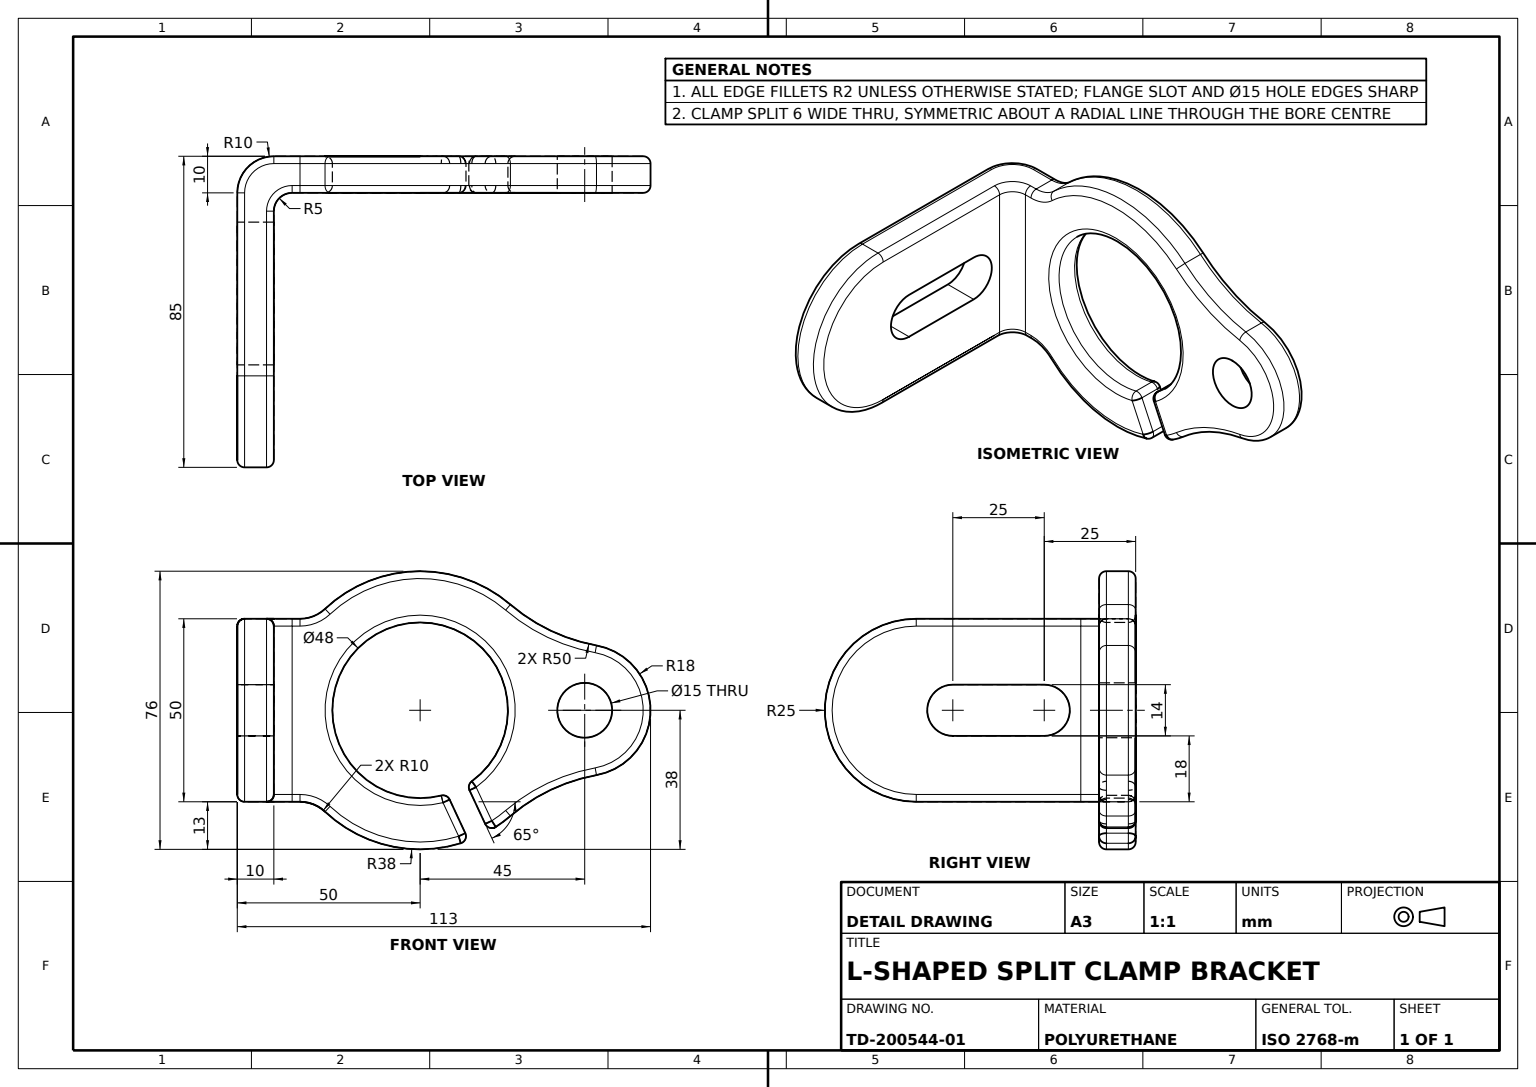
solid
v1 (-28.889805,-74.685606,8)
v2 (-28.889805,-74.685606,2)
e1 v1 v2 LINE
v3 (-38,-50,8)
e2 v1 v3 CIRCLE(AX(P(0,-50,8),D(0,0,-1),D(1,0,0)),38)
v4 (-38,-50,2)
e3 v3 v4 LINE
e4 v4 v2 CIRCLE(AX(P(0,-50,2),D(0,0,1),D(1,0,0)),38)
face CYL(AX(P(0,-50,10),D(0,0,-1),D(-1,0,0)),38) [-e1 e2 e3 e4]
v5 (-23,-10,-50)
v6 (-25,-8,-50)
e5 v5 v6 CIRCLE(AX(P(-23,-8,-50),D(0,0,-1),D(-1,0,0)),2)
v7 (25,-8,-50)
e6 v7 v6 CIRCLE(AX(P(0,-8,-50),D(0,1,0),D(1,0,0)),25)
v8 (23,-10,-50)
e7 v8 v7 CIRCLE(AX(P(23,-8,-50),D(0,0,1),D(1,0,0)),2)
e8 v5 v8 CIRCLE(AX(P(0,-10,-50),D(0,-1,0),D(1,0,0)),23)
face TORUS(AX(P(0,-8,-50),D(0,-1,0),D(1,0,0)),23,2) [e5 -e6 -e7 -e8]
v9 (26,-50,10)
v10 (24,-50,8)
e9 v9 v10 CIRCLE(AX(P(26,-50,8),D(0,-1,0),D(0,0,-1)),2)
v11 (-26,-50,10)
e10 v11 v9 CIRCLE(AX(P(0,-50,10),D(0,0,-1),D(1,0,0)),26)
v12 (-24,-50,8)
e11 v11 v12 CIRCLE(AX(P(-26,-50,8),D(0,1,0),D(-1,0,0)),2)
e12 v10 v12 CIRCLE(AX(P(0,-50,8),D(0,0,1),D(1,0,0)),24)
face TORUS(AX(P(0,-50,8),D(0,0,1),D(1,0,0)),26,2) [-e9 -e10 e11 -e12]
v13 (23.295936,-55.77056,2)
v14 (23.237264,-56.25144,2)
e13 v13 v14 CIRCLE(AX(P(25.237264,-56.25144,2),D(0,0,1),D(-1,0,0)),2)
v15 (23.237264,-56.25144,8)
e14 v15 v14 LINE
v16 (23.295936,-55.77056,8)
e15 v16 v15 CIRCLE(AX(P(25.237264,-56.25144,8),D(0,0,1),D(1,0,0)),2)
e16 v13 v16 LINE
face CYL(AX(P(25.237264,-56.25144,10),D(0,0,-1),D(-1,0,0)),2) [e13 -e14 -e15 -e16]
v17 (-25,-2,-50)
v18 (25,-2,-50)
e17 v17 v18 CIRCLE(AX(P(0,-2,-50),D(0,-1,0),D(1,0,0)),25)
v19 (-23,0,-50)
e18 v19 v17 CIRCLE(AX(P(-23,-2,-50),D(0,0,1),D(1,0,0)),2)
v20 (23,0,-50)
e19 v20 v19 CIRCLE(AX(P(0,0,-50),D(0,1,0),D(1,0,0)),23)
e20 v20 v18 CIRCLE(AX(P(23,-2,-50),D(0,0,-1),D(-1,0,0)),2)
face TORUS(AX(P(0,-2,-50),D(0,-1,0),D(1,0,0)),23,2) [-e17 -e18 -e19 e20]
v21 (-7.5,-95,0)
v22 (7.5,-95,0)
e21 v21 v22 CIRCLE(AX(P(0,-95,0),D(0,0,1),D(1,0,0)),7.5)
v23 (-7.5,-95,10)
e22 v23 v21 LINE
v24 (7.5,-95,10)
e23 v23 v24 CIRCLE(AX(P(0,-95,10),D(0,0,1),D(1,0,0)),7.5)
e24 v24 v22 LINE
face CYL(AX(P(0,-95,10),D(0,0,-1),D(-1,0,0)),7.5) rev [-e21 -e22 e23 e24]
v25 (17.70954,-98.220588,8)
v26 (15.741813,-97.862745,10)
e25 v25 v26 CIRCLE(AX(P(15.741813,-97.862745,8),D(-0.178921569,-0.98386334,0),D(0.98386334,-0.178921569,0)),2)
v27 (-15.741813,-97.862745,10)
e26 v27 v26 CIRCLE(AX(P(0,-95,10),D(0,0,1),D(1,0,0)),16)
v28 (-17.70954,-98.220588,8)
e27 v28 v27 CIRCLE(AX(P(-15.741813,-97.862745,8),D(-0.178921569,0.98386334,0),D(-0.98386334,-0.178921569,0)),2)
e28 v25 v28 CIRCLE(AX(P(0,-95,8),D(0,0,-1),D(1,0,0)),18)
face TORUS(AX(P(0,-95,8),D(0,0,1),D(1,0,0)),16,2) [e25 -e26 -e27 -e28]
v29 (23,-10,10)
v30 (-23,-10,10)
e29 v29 v30 LINE
v31 (23,0,0)
e30 v29 v31 CIRCLE(AX(P(23,-10,0),D(-1,0,0),D(0,-1,0)),10)
v32 (-23,0,0)
e31 v32 v31 LINE
e32 v32 v30 CIRCLE(AX(P(-23,-10,0),D(1,0,0),D(0,1,0)),10)
face CYL(AX(P(-66.902707,-10,0),D(1,0,0),D(0,1,0)),10) [-e29 e30 -e31 e32]
v33 (28.889805,-74.685606,2)
v34 (27.369289,-73.386364,0)
e33 v33 v34 CIRCLE(AX(P(27.369289,-73.386364,2),D(0.649621212,0.760258036,0),D(-0.760258036,0.649621212,0)),2)
v35 (17.70954,-98.220588,2)
e34 v35 v33 CIRCLE(AX(P(66.902707,-107.166667,2),D(0,0,-1),D(1,0,0)),50)
v36 (15.741813,-97.862745,0)
e35 v35 v36 CIRCLE(AX(P(15.741813,-97.862745,2),D(0.178921569,0.98386334,0),D(-0.98386334,0.178921569,0)),2)
e36 v34 v36 CIRCLE(AX(P(66.902707,-107.166667,0),D(0,0,1),D(1,0,0)),52)
face TORUS(AX(P(66.902707,-107.166667,2),D(0,0,1),D(1,0,0)),52,2) [-e33 -e34 e35 -e36]
v37 (19.394844,-64.136478,8)
v38 (19.394844,-64.136478,2)
e37 v37 v38 LINE
v39 (21.856318,-63.501902,8)
e38 v39 v37 CIRCLE(AX(P(21.011081,-65.314518,8),D(0,0,1),D(1,0,0)),2)
v40 (21.856318,-63.501902,2)
e39 v40 v39 LINE
v41 (21.011081,-63.314518,2)
e40 v40 v41 CIRCLE(AX(P(21.011081,-65.314518,2),D(0,0,1),D(-1,0,0)),2)
e41 v41 v38 CIRCLE(AX(P(21.011081,-65.314518,2),D(0,0,1),D(-1,0,0)),2)
face CYL(AX(P(21.011081,-65.314518,10),D(0,0,-1),D(-1,0,0)),2) [-e37 -e38 -e39 e40 e41]
v42 (-25,-10,8)
e42 v30 v42 CIRCLE(AX(P(-23,-10,8),D(0,-1,0),D(0,0,-1)),2)
v43 (-25,-17.151865,8)
e43 v43 v42 LINE
v44 (-23,-17.151865,10)
e44 v43 v44 CIRCLE(AX(P(-23,-17.151865,8),D(0,1,0),D(0,0,1)),2)
e45 v30 v44 LINE
face CYL(AX(P(-23,-107.166667,8),D(0,1,0),D(-1,0,0)),2) [e42 -e43 e44 -e45]
v45 (-17.70954,-98.220588,2)
e46 v45 v35 CIRCLE(AX(P(0,-95,2),D(0,0,1),D(1,0,0)),18)
v46 (-15.741813,-97.862745,0)
e47 v45 v46 CIRCLE(AX(P(-15.741813,-97.862745,2),D(0.178921569,-0.98386334,0),D(0.98386334,0.178921569,0)),2)
e48 v36 v46 CIRCLE(AX(P(0,-95,0),D(0,0,-1),D(1,0,0)),16)
face TORUS(AX(P(0,-95,2),D(0,0,1),D(1,0,0)),16,2) [-e46 e47 -e48 -e35]
v47 (31.87542,-70.687136,2)
v48 (30.197766,-69.598339,0)
e49 v47 v48 CIRCLE(AX(P(30.197766,-69.598339,2),D(0.544398315,0.838826844,0),D(-0.838826844,0.544398315,0)),2)
v49 (31.043003,-67.785724,2)
e50 v48 v49 CIRCLE(AX(P(30.197766,-69.598339,2),D(0.906307787,-0.422618262,0),D(0.422618262,0.906307787,0)),2)
e51 v47 v49 CIRCLE(AX(P(30.197766,-69.598339,2),D(0,0,1),D(-1,0,0)),2)
face SPHERE(AX(P(30.197766,-69.598339,2),D(0,1,0),D(-1,0,0)),2) [e49 e50 -e51]
v50 (-25,-2,0)
e52 v50 v17 LINE
e53 v32 v50 CIRCLE(AX(P(-23,-2,0),D(0,0,1),D(1,0,0)),2)
e54 v19 v32 LINE
face CYL(AX(P(-23,-2,10),D(0,0,-1),D(-1,0,0)),2) [-e52 -e53 -e54 e18]
e55 v33 v47 CIRCLE(AX(P(0,-50,2),D(0,0,1),D(1,0,0)),38)
e56 v48 v34 CIRCLE(AX(P(0,-50,0),D(0,0,-1),D(1,0,0)),36)
face TORUS(AX(P(0,-50,2),D(0,0,1),D(1,0,0)),36,2) [-e55 e33 -e56 -e49]
v51 (7,-10,-40)
v52 (7,0,-40)
e57 v51 v52 LINE
v53 (-7,0,-40)
e58 v52 v53 CIRCLE(AX(P(0,0,-40),D(0,1,0),D(-1,0,0)),7)
v54 (-7,-10,-40)
e59 v54 v53 LINE
e60 v51 v54 CIRCLE(AX(P(0,-10,-40),D(0,1,0),D(-1,0,0)),7)
face CYL(AX(P(0,-10,-40),D(0,1,0),D(-1,0,0)),7) rev [e57 e58 -e59 -e60]
v55 (-24,-50,2)
e61 v38 v55 CIRCLE(AX(P(0,-50,2),D(0,0,-1),D(1,0,0)),24)
e62 v12 v55 LINE
e63 v12 v37 CIRCLE(AX(P(0,-50,8),D(0,0,1),D(1,0,0)),24)
face CYL(AX(P(0,-50,10),D(0,0,-1),D(-1,0,0)),24) rev [e61 -e62 e63 e37]
v56 (7,-10,-15)
e64 v56 v51 LINE
v57 (7,0,-15)
e65 v56 v57 LINE
e66 v57 v52 LINE
face PLANE(AX(P(7,-10,-40),D(1,0,0),D(0,0,-1))) rev [-e64 e65 e66 -e57]
v58 (25.237264,-56.25144,10)
v59 (24.392028,-58.064055,8)
e67 v58 v59 CIRCLE(AX(P(25.237264,-56.25144,8),D(0.906307787,-0.422618262,0),D(-0.422618262,-0.906307787,0)),2)
e68 v16 v58 CIRCLE(AX(P(25.237264,-56.25144,8),D(0.240439997,0.970664004,0),D(0.970664004,-0.240439997,0)),2)
e69 v15 v59 CIRCLE(AX(P(25.237264,-56.25144,8),D(0,0,1),D(1,0,0)),2)
face SPHERE(AX(P(25.237264,-56.25144,8),D(1,0,0),D(0,-1,0)),2) [-e67 -e68 e15 e69]
v60 (23,-10,-5)
e70 v8 v60 LINE
v61 (25,-8,-5)
e71 v61 v7 LINE
e72 v60 v61 CIRCLE(AX(P(23,-8,-5),D(0,0,1),D(1,0,0)),2)
face CYL(AX(P(23,-8,10),D(0,0,1),D(1,0,0)),2) [-e70 e7 -e71 -e72]
v62 (25,-17.151865,8)
v63 (27.708333,-23.995226,8)
e73 v62 v63 CIRCLE(AX(P(35,-17.151865,8),D(0,0,1),D(1,0,0)),10)
v64 (23,-17.151865,10)
e74 v64 v62 CIRCLE(AX(P(23,-17.151865,8),D(0,1,0),D(0,0,1)),2)
v65 (26.25,-25.363898,10)
e75 v65 v64 CIRCLE(AX(P(35,-17.151865,10),D(0,0,-1),D(1,0,0)),12)
e76 v65 v63 CIRCLE(AX(P(26.25,-25.363898,8),D(-0.684336154,0.729166667,0),D(-0.729166667,-0.684336154,0)),2)
face TORUS(AX(P(35,-17.151865,8),D(0,0,1),D(1,0,0)),12,2) [-e73 -e74 -e75 e76]
e77 v28 v45 LINE
e78 v25 v35 LINE
face CYL(AX(P(0,-95,10),D(0,0,-1),D(-1,0,0)),18) [e28 e77 e46 -e78]
v66 (-7,-10,-15)
e79 v54 v66 LINE
e80 v66 v56 CIRCLE(AX(P(0,-10,-15),D(0,1,0),D(-1,0,0)),7)
v67 (-23,-10,-5)
e81 v67 v5 LINE
e82 v60 v67 LINE
face PLANE(AX(P(0,-10,-50),D(0,-1,0),D(1,0,0))) [e79 e80 e64 e60] [e81 e8 e70 e82]
e83 v42 v50 CIRCLE(AX(P(-25,-10,0),D(-1,0,0),D(0,1,0)),8)
e84 v6 v17 LINE
v68 (-25,-8,-5)
e85 v6 v68 LINE
v69 (-25,-15,2)
e86 v68 v69 CIRCLE(AX(P(-25,-15,-5),D(1,0,0),D(0,1,0)),7)
v70 (-25,-17.151865,2)
e87 v69 v70 LINE
e88 v43 v70 LINE
face PLANE(AX(P(-25,0,10),D(1,0,0),D(0,1,0))) rev [e43 e83 e52 -e84 e85 e86 e87 -e88]
v71 (24,-50,2)
e89 v71 v13 CIRCLE(AX(P(0,-50,2),D(0,0,-1),D(1,0,0)),24)
e90 v16 v10 CIRCLE(AX(P(0,-50,8),D(0,0,1),D(1,0,0)),24)
e91 v10 v71 LINE
face CYL(AX(P(0,-50,10),D(0,0,-1),D(-1,0,0)),24) rev [e89 e16 e90 e91]
v72 (25,-2,0)
e92 v18 v72 LINE
v73 (25,-10,8)
e93 v72 v73 CIRCLE(AX(P(25,-10,0),D(1,0,0),D(0,-1,0)),8)
e94 v73 v62 LINE
v74 (25,-17.151865,2)
e95 v62 v74 LINE
v75 (25,-15,2)
e96 v74 v75 LINE
e97 v75 v61 CIRCLE(AX(P(25,-15,-5),D(-1,0,0),D(0,-1,0)),7)
e98 v7 v18 LINE
face PLANE(AX(P(25,0,10),D(-1,0,0),D(0,-1,0))) rev [e92 e93 e94 e95 e96 e97 e71 e98]
e99 v9 v58 CIRCLE(AX(P(0,-50,10),D(0,0,-1),D(1,0,0)),26)
face TORUS(AX(P(0,-50,8),D(0,0,1),D(1,0,0)),26,2) [e68 -e99 e9 -e90]
v76 (31.043003,-67.785724,8)
e100 v39 v76 LINE
e101 v76 v49 LINE
e102 v49 v40 LINE
face PLANE(AX(P(35.208422,-69.728091,10),D(-0.422618262,-0.906307787,0),D(0.906307787,-0.422618262,0))) rev [e39 e100 e101 e102]
e103 v29 v73 CIRCLE(AX(P(23,-10,8),D(0,1,0),D(0,0,1)),2)
e104 v64 v29 LINE
face CYL(AX(P(23,-107.166667,8),D(0,-1,0),D(1,0,0)),2) [e74 -e94 -e103 -e104]
v77 (-27.369289,-73.386364,10)
e105 v1 v77 CIRCLE(AX(P(-27.369289,-73.386364,8),D(-0.649621212,0.760258036,0),D(-0.760258036,-0.649621212,0)),2)
e106 v28 v1 CIRCLE(AX(P(-66.902707,-107.166667,8),D(0,0,1),D(1,0,0)),50)
e107 v77 v27 CIRCLE(AX(P(-66.902707,-107.166667,10),D(0,0,-1),D(1,0,0)),52)
face TORUS(AX(P(-66.902707,-107.166667,8),D(0,0,1),D(1,0,0)),52,2) [-e105 -e106 e27 -e107]
e108 v55 v71 CIRCLE(AX(P(0,-50,2),D(0,0,-1),D(1,0,0)),24)
v78 (-26,-50,0)
e109 v55 v78 CIRCLE(AX(P(-26,-50,2),D(0,1,0),D(-1,0,0)),2)
v79 (26,-50,0)
e110 v79 v78 CIRCLE(AX(P(0,-50,0),D(0,0,1),D(1,0,0)),26)
e111 v71 v79 CIRCLE(AX(P(26,-50,2),D(0,-1,0),D(0,0,-1)),2)
face TORUS(AX(P(0,-50,2),D(0,0,1),D(1,0,0)),26,2) [-e108 e109 -e110 -e111]
e112 v24 v23 CIRCLE(AX(P(0,-95,10),D(0,0,1),D(1,0,0)),7.5)
v80 (-26.25,-25.363898,10)
e113 v44 v80 CIRCLE(AX(P(-35,-17.151865,10),D(0,0,-1),D(1,0,0)),12)
e114 v80 v77 CIRCLE(AX(P(0,-50,10),D(0,0,1),D(1,0,0)),36)
v81 (27.369289,-73.386364,10)
e115 v26 v81 CIRCLE(AX(P(66.902707,-107.166667,10),D(0,0,-1),D(1,0,0)),52)
v82 (30.197766,-69.598339,10)
e116 v81 v82 CIRCLE(AX(P(0,-50,10),D(0,0,1),D(1,0,0)),36)
v83 (21.011081,-65.314518,10)
e117 v82 v83 LINE
e118 v83 v11 CIRCLE(AX(P(0,-50,10),D(0,0,-1),D(1,0,0)),26)
v84 (34.423949,-60.535261,10)
e119 v58 v84 LINE
v85 (36,-50,10)
e120 v84 v85 CIRCLE(AX(P(0,-50,10),D(0,0,1),D(1,0,0)),36)
e121 v85 v65 CIRCLE(AX(P(0,-50,10),D(0,0,1),D(1,0,0)),36)
face PLANE(AX(P(-66.902707,-107.166667,10),D(0,0,1),D(1,0,0))) [-e23 -e112] [e45 e113 e114 e107 e26 e115 e116 e117 e118 e10 e99 e119 e120 e121 e75 e104 e29]
v86 (31.87542,-70.687136,8)
e122 v86 v76 CIRCLE(AX(P(30.197766,-69.598339,8),D(0,0,1),D(1,0,0)),2)
e123 v76 v82 CIRCLE(AX(P(30.197766,-69.598339,8),D(0.906307787,-0.422618262,0),D(0.422618262,0.906307787,0)),2)
e124 v86 v82 CIRCLE(AX(P(30.197766,-69.598339,8),D(-0.544398315,-0.838826844,0),D(-0.838826844,0.544398315,0)),2)
face SPHERE(AX(P(30.197766,-69.598339,8),D(1,0,0),D(0,-1,0)),2) [e122 e123 -e124]
e125 v47 v86 LINE
face CYL(AX(P(30.197766,-69.598339,10),D(0,0,-1),D(-1,0,0)),2) [-e101 -e122 -e125 e51]
v87 (24.392028,-58.064055,2)
v88 (33.578712,-62.347877,2)
e126 v87 v88 LINE
v89 (33.578712,-62.347877,8)
e127 v88 v89 LINE
e128 v89 v59 LINE
e129 v59 v87 LINE
face PLANE(AX(P(37.744132,-64.290244,10),D(0.422618262,0.906307787,0),D(-0.906307787,0.422618262,0))) rev [e126 e127 e128 e129]
v90 (28.889805,-74.685606,8)
e130 v90 v81 CIRCLE(AX(P(27.369289,-73.386364,8),D(-0.649621212,-0.760258036,0),D(0.760258036,-0.649621212,0)),2)
e131 v86 v90 CIRCLE(AX(P(0,-50,8),D(0,0,-1),D(1,0,0)),38)
face TORUS(AX(P(0,-50,8),D(0,0,1),D(1,0,0)),36,2) [-e130 -e131 e124 -e116]
v91 (27.708333,-23.995226,2)
e132 v91 v74 CIRCLE(AX(P(35,-17.151865,2),D(0,0,-1),D(1,0,0)),10)
e133 v63 v91 LINE
face CYL(AX(P(35,-17.151865,10),D(0,0,-1),D(-1,0,0)),10) rev [e132 -e95 e73 e133]
v92 (-23,-17.151865,0)
e134 v70 v92 CIRCLE(AX(P(-23,-17.151865,2),D(0,-1,0),D(0,0,-1)),2)
v93 (-26.25,-25.363898,0)
e135 v93 v92 CIRCLE(AX(P(-35,-17.151865,0),D(0,0,1),D(1,0,0)),12)
v94 (-27.708333,-23.995226,2)
e136 v94 v93 CIRCLE(AX(P(-26.25,-25.363898,2),D(-0.684336154,-0.729166667,0),D(0.729166667,-0.684336154,0)),2)
e137 v70 v94 CIRCLE(AX(P(-35,-17.151865,2),D(0,0,-1),D(1,0,0)),10)
face TORUS(AX(P(-35,-17.151865,2),D(0,0,1),D(1,0,0)),12,2) [e134 -e135 -e136 -e137]
v95 (-23,-15,0)
v96 (23,-15,0)
e138 v95 v96 LINE
v97 (23,-17.151865,0)
e139 v96 v97 LINE
v98 (26.25,-25.363898,0)
e140 v97 v98 CIRCLE(AX(P(35,-17.151865,0),D(0,0,1),D(1,0,0)),12)
v99 (36,-50,0)
e141 v98 v99 CIRCLE(AX(P(0,-50,0),D(0,0,-1),D(1,0,0)),36)
v100 (34.423949,-60.535261,0)
e142 v99 v100 CIRCLE(AX(P(0,-50,0),D(0,0,-1),D(1,0,0)),36)
v101 (25.237264,-56.25144,0)
e143 v100 v101 LINE
e144 v101 v79 CIRCLE(AX(P(0,-50,0),D(0,0,1),D(1,0,0)),26)
v102 (21.011081,-65.314518,0)
e145 v78 v102 CIRCLE(AX(P(0,-50,0),D(0,0,1),D(1,0,0)),26)
e146 v102 v48 LINE
v103 (-27.369289,-73.386364,0)
e147 v46 v103 CIRCLE(AX(P(-66.902707,-107.166667,0),D(0,0,1),D(1,0,0)),52)
e148 v103 v93 CIRCLE(AX(P(0,-50,0),D(0,0,-1),D(1,0,0)),36)
e149 v92 v95 LINE
e150 v22 v21 CIRCLE(AX(P(0,-95,0),D(0,0,1),D(1,0,0)),7.5)
face PLANE(AX(P(-66.902707,-107.166667,0),D(0,0,1),D(1,0,0))) rev [e138 e139 e140 e141 e142 e143 e144 e110 e145 e146 e56 e36 e48 e147 e148 e135 e149] [e150 e21]
e151 v87 v101 CIRCLE(AX(P(25.237264,-56.25144,2),D(0.906307787,-0.422618262,0),D(-0.422618262,-0.906307787,0)),2)
e152 v14 v87 CIRCLE(AX(P(25.237264,-56.25144,2),D(0,0,1),D(-1,0,0)),2)
e153 v14 v101 CIRCLE(AX(P(25.237264,-56.25144,2),D(0,-1,0),D(0,0,-1)),2)
face SPHERE(AX(P(25.237264,-56.25144,2),D(0,1,0),D(-1,0,0)),2) [-e151 -e152 e153]
v104 (36.336391,-61.120554,8)
e154 v84 v104 CIRCLE(AX(P(34.423949,-60.535261,8),D(0.292646152,0.956220806,0),D(0.956220806,-0.292646152,0)),2)
v105 (34.423949,-62.535261,8)
e155 v105 v84 CIRCLE(AX(P(34.423949,-60.535261,8),D(-1,0,0),D(0,0,1)),2)
e156 v105 v104 CIRCLE(AX(P(34.423949,-60.535261,8),D(0,0,1),D(1,0,0)),2)
face SPHERE(AX(P(34.423949,-60.535261,8),D(1,0,0),D(0,-1,0)),2) [-e154 -e155 e156]
v106 (36.336391,-61.120554,2)
v107 (38,-50,2)
e157 v106 v107 CIRCLE(AX(P(0,-50,2),D(0,0,1),D(1,0,0)),38)
e158 v100 v106 CIRCLE(AX(P(34.423949,-60.535261,2),D(-0.292646152,-0.956220806,0),D(0.956220806,-0.292646152,0)),2)
e159 v99 v107 CIRCLE(AX(P(36,-50,2),D(0,-1,0),D(0,0,-1)),2)
face TORUS(AX(P(0,-50,2),D(0,0,1),D(1,0,0)),36,2) [-e157 -e158 -e142 e159]
e160 v88 v100 CIRCLE(AX(P(34.423949,-60.535261,2),D(0.906307787,-0.422618262,0),D(0.422618262,0.906307787,0)),2)
face CYL(AX(P(38.589368,-62.477628,2),D(0.906307787,-0.422618262,0),D(0.422618262,0.906307787,0)),2) [-e160 -e126 e151 -e143]
e161 v102 v38 CIRCLE(AX(P(21.011081,-65.314518,2),D(0.589019915,0.808118518,0),D(-0.808118518,0.589019915,0)),2)
face TORUS(AX(P(0,-50,2),D(0,0,1),D(1,0,0)),26,2) [-e61 -e161 -e145 -e109]
e162 v90 v25 CIRCLE(AX(P(66.902707,-107.166667,8),D(0,0,1),D(1,0,0)),50)
face TORUS(AX(P(66.902707,-107.166667,8),D(0,0,1),D(1,0,0)),52,2) [-e25 -e162 e130 -e115]
e163 v2 v45 CIRCLE(AX(P(-66.902707,-107.166667,2),D(0,0,-1),D(1,0,0)),50)
e164 v2 v103 CIRCLE(AX(P(-27.369289,-73.386364,2),D(0.649621212,-0.760258036,0),D(0.760258036,0.649621212,0)),2)
face TORUS(AX(P(-66.902707,-107.166667,2),D(0,0,1),D(1,0,0)),52,2) [-e47 -e163 e164 -e147]
e165 v31 v72 CIRCLE(AX(P(23,-2,0),D(0,0,-1),D(-1,0,0)),2)
face TORUS(AX(P(23,-10,0),D(-1,0,0),D(0,-1,0)),8,2) [-e30 e103 -e93 -e165]
v108 (38,-50,8)
e166 v108 v85 CIRCLE(AX(P(36,-50,8),D(0,-1,0),D(0,0,-1)),2)
e167 v63 v108 CIRCLE(AX(P(0,-50,8),D(0,0,-1),D(1,0,0)),38)
face TORUS(AX(P(0,-50,8),D(0,0,1),D(1,0,0)),36,2) [-e166 -e167 -e76 -e121]
e168 v84 v89 CIRCLE(AX(P(34.423949,-60.535261,8),D(0.906307787,-0.422618262,0),D(0.422618262,0.906307787,0)),2)
face CYL(AX(P(-30.944274,-30.053558,8),D(-0.906307787,0.422618262,0),D(-0.422618262,-0.906307787,0)),2) [e67 -e128 -e168 -e119]
e169 v94 v4 CIRCLE(AX(P(0,-50,2),D(0,0,1),D(1,0,0)),38)
v109 (-27.708333,-23.995226,8)
e170 v3 v109 CIRCLE(AX(P(0,-50,8),D(0,0,-1),D(1,0,0)),38)
e171 v109 v94 LINE
face CYL(AX(P(0,-50,10),D(0,0,-1),D(-1,0,0)),38) [e169 -e3 e170 e171]
e172 v108 v104 CIRCLE(AX(P(0,-50,8),D(0,0,-1),D(1,0,0)),38)
face TORUS(AX(P(0,-50,8),D(0,0,1),D(1,0,0)),36,2) [e154 -e172 e166 -e120]
e173 v68 v67 CIRCLE(AX(P(-23,-8,-5),D(0,0,1),D(0,-1,0)),2)
face CYL(AX(P(-23,-8,10),D(0,0,-1),D(-1,0,0)),2) [-e81 -e173 -e85 -e5]
e174 v37 v83 CIRCLE(AX(P(21.011081,-65.314518,8),D(0.589019915,0.808118518,0),D(-0.808118518,0.589019915,0)),2)
e175 v39 v83 CIRCLE(AX(P(21.011081,-65.314518,8),D(0.906307787,-0.422618262,0),D(-0.422618262,-0.906307787,0)),2)
face SPHERE(AX(P(21.011081,-65.314518,8),D(0,1,0),D(1,0,0)),2) [e38 e174 -e175]
face TORUS(AX(P(0,-50,2),D(0,0,1),D(1,0,0)),36,2) [e136 -e148 -e164 -e4 -e169]
e176 v109 v43 CIRCLE(AX(P(-35,-17.151865,8),D(0,0,1),D(1,0,0)),10)
face CYL(AX(P(-35,-17.151865,10),D(0,0,-1),D(-1,0,0)),10) rev [e176 e88 e137 -e171]
e177 v95 v67 CIRCLE(AX(P(-23,-15,-5),D(-1,0,0),D(0,1,0)),5)
e178 v69 v95 CIRCLE(AX(P(-23,-15,2),D(0,-1,0),D(0,0,-1)),2)
face TORUS(AX(P(-23,-15,-5),D(1,0,0),D(0,1,0)),7,2) [-e86 e173 -e177 -e178]
e179 v96 v75 CIRCLE(AX(P(23,-15,2),D(0,-1,0),D(0,0,-1)),2)
e180 v97 v74 CIRCLE(AX(P(23,-17.151865,2),D(0,-1,0),D(0,0,-1)),2)
face CYL(AX(P(23,0,2),D(0,1,0),D(-1,0,0)),2) [-e139 e179 -e96 -e180]
e181 v102 v40 CIRCLE(AX(P(21.011081,-65.314518,2),D(0.906307787,-0.422618262,0),D(-0.422618262,-0.906307787,0)),2)
face CYL(AX(P(34.363186,-71.540706,2),D(-0.906307787,0.422618262,0),D(-0.422618262,-0.906307787,0)),2) [-e146 e181 -e102 -e50]
v110 (-7,0,-15)
e182 v66 v110 LINE
e183 v110 v57 CIRCLE(AX(P(0,0,-15),D(0,1,0),D(-1,0,0)),7)
face CYL(AX(P(0,-10,-15),D(0,1,0),D(-1,0,0)),7) rev [e182 e183 -e65 -e80]
e184 v90 v33 LINE
face CYL(AX(P(66.902707,-107.166667,10),D(0,0,-1),D(-1,0,0)),50) rev [-e184 e162 e78 e34]
e185 v109 v80 CIRCLE(AX(P(-26.25,-25.363898,8),D(0.684336154,0.729166667,0),D(-0.729166667,0.684336154,0)),2)
face TORUS(AX(P(0,-50,8),D(0,0,1),D(1,0,0)),36,2) [-e114 -e185 -e170 -e2 e105]
e186 v31 v20 LINE
face CYL(AX(P(23,-2,10),D(0,0,-1),D(-1,0,0)),2) [-e186 e165 -e92 -e20]
face CYL(AX(P(-23,0,2),D(0,-1,0),D(1,0,0)),2) [-e134 -e87 e178 -e149]
face CYL(AX(P(-66.902707,-107.166667,10),D(0,0,-1),D(-1,0,0)),50) rev [e106 e1 e163 -e77]
face CYL(AX(P(0,-10,-50),D(0,1,0),D(-1,0,0)),25) [e84 e17 -e98 e6]
e187 v98 v91 CIRCLE(AX(P(26.25,-25.363898,2),D(0.684336154,-0.729166667,0),D(0.729166667,0.684336154,0)),2)
e188 v107 v91 CIRCLE(AX(P(0,-50,2),D(0,0,1),D(1,0,0)),38)
face TORUS(AX(P(0,-50,2),D(0,0,1),D(1,0,0)),36,2) [e187 -e188 -e159 -e141]
e189 v89 v105 CIRCLE(AX(P(34.423949,-60.535261,8),D(0,0,1),D(1,0,0)),2)
face SPHERE(AX(P(34.423949,-60.535261,8),D(1,0,0),D(0,-1,0)),2) [e189 e155 e168]
face CYL(AX(P(-35.170457,-39.116636,8),D(0.906307787,-0.422618262,0),D(0.422618262,0.906307787,0)),2) [e175 -e117 -e123 -e100]
face CYL(AX(P(0,-50,10),D(0,0,-1),D(-1,0,0)),24) rev [e108 -e91 e12 e62]
e190 v41 v102 CIRCLE(AX(P(21.011081,-65.314518,2),D(-1,0,0),D(0,0,1)),2)
face SPHERE(AX(P(21.011081,-65.314518,2),D(1,0,0),D(0,1,0)),2) [-e40 -e181 -e190]
e191 v88 v106 CIRCLE(AX(P(34.423949,-60.535261,2),D(0,0,1),D(-1,0,0)),2)
e192 v104 v106 LINE
face CYL(AX(P(34.423949,-60.535261,10),D(0,0,-1),D(-1,0,0)),2) [e191 -e192 -e156 -e189 -e127]
face SPHERE(AX(P(21.011081,-65.314518,2),D(1,0,0),D(0,1,0)),2) [e190 e161 -e41]
e193 v53 v110 LINE
face PLANE(AX(P(25,0,10),D(0,-1,0),D(1,0,0))) rev [e186 e19 e54 e31] [-e58 -e66 -e183 -e193]
face CYL(AX(P(0,-95,10),D(0,0,-1),D(-1,0,0)),7.5) rev [e22 -e150 -e24 e112]
face CYL(AX(P(0,-50,10),D(0,0,-1),D(-1,0,0)),38) [e184 e55 e125 e131]
face CYL(AX(P(0,-50,10),D(0,0,-1),D(-1,0,0)),38) [e167 e172 e192 e157 e188 -e133]
e194 v60 v96 CIRCLE(AX(P(23,-15,-5),D(1,0,0),D(0,-1,0)),5)
face TORUS(AX(P(23,-15,-5),D(-1,0,0),D(0,-1,0)),7,2) [-e194 e72 -e97 -e179]
face TORUS(AX(P(35,-17.151865,2),D(0,0,1),D(1,0,0)),12,2) [-e140 e180 -e132 -e187]
face CYL(AX(P(-66.902707,-15,-5),D(1,0,0),D(0,1,0)),5) rev [e177 -e82 e194 -e138]
face PLANE(AX(P(-7,-10,-40),D(-1,0,0),D(0,0,1))) rev [e193 -e182 -e79 e59]
face TORUS(AX(P(0,-50,8),D(0,0,1),D(1,0,0)),26,2) [-e118 -e174 -e63 -e11]
face SPHERE(AX(P(34.423949,-60.535261,2),D(1,0,0),D(0,1,0)),2) [e158 -e191 e160]
face CYL(AX(P(25.237264,-56.25144,10),D(0,0,-1),D(-1,0,0)),2) [e14 e152 -e129 -e69]
e195 v101 v13 CIRCLE(AX(P(25.237264,-56.25144,2),D(0.240439997,0.970664004,0),D(0.970664004,-0.240439997,0)),2)
face SPHERE(AX(P(25.237264,-56.25144,2),D(0,1,0),D(-1,0,0)),2) [-e13 -e195 -e153]
face TORUS(AX(P(0,-50,2),D(0,0,1),D(1,0,0)),26,2) [e111 -e144 e195 -e89]
face TORUS(AX(P(-23,-10,0),D(1,0,0),D(0,1,0)),8,2) [-e83 -e42 -e32 e53]
face TORUS(AX(P(-35,-17.151865,8),D(0,0,1),D(1,0,0)),12,2) [-e113 -e44 -e176 e185]
